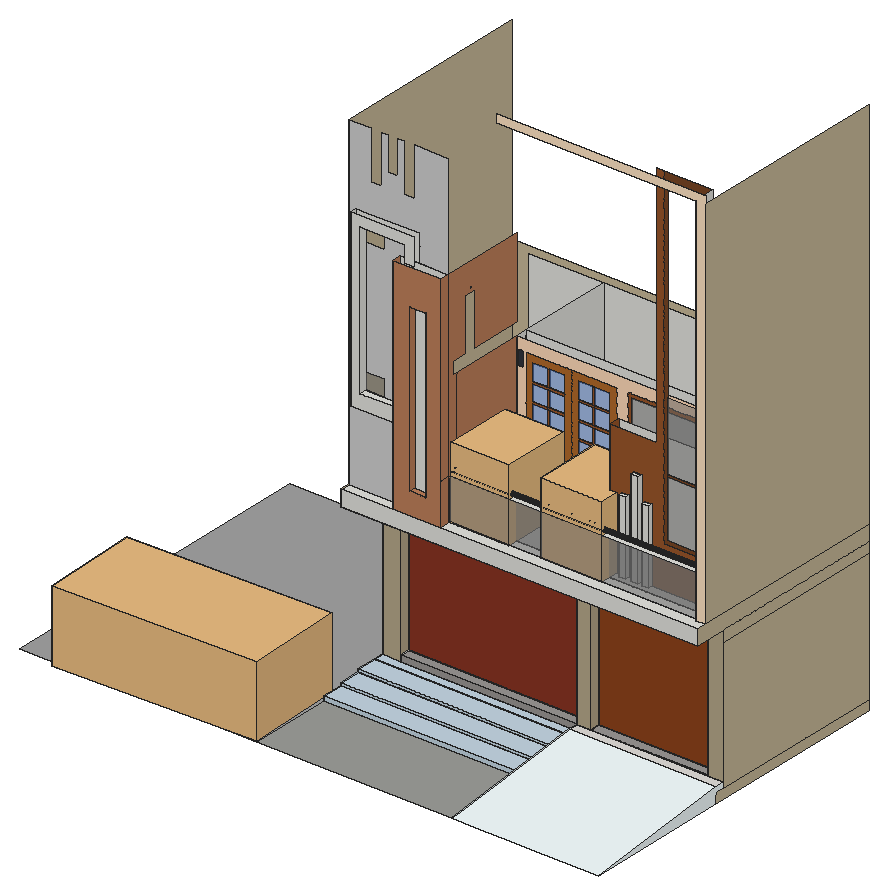
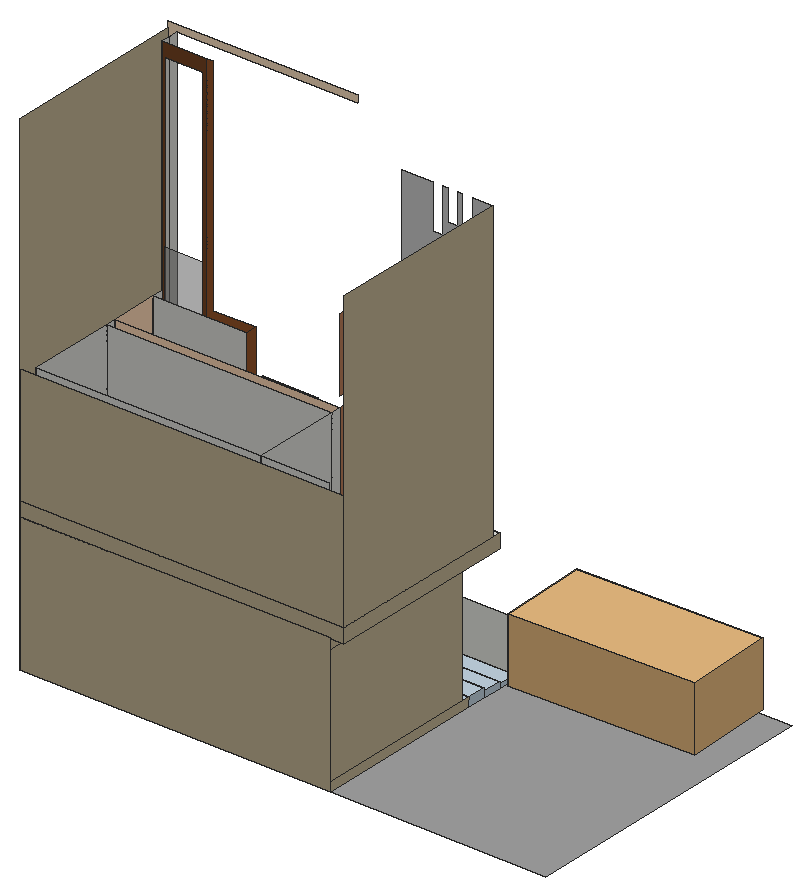
# SketchUp Ruby script. Lengths in inches.
U = 1.inch
M = Sketchup.active_model
def pt(a) = Geom::Point3d.new(a.map { |v| v * U })
def face(e, loops, mat)
  f = e.add_face(loops[0].map { |a| pt(a) })
  loops[1..].each { |l| e.add_face(l.map { |a| pt(a) }).erase! }
  f.material = f.back_material = mat if mat
  f
end
# faces: each face lists its corners as indices into pts; further lists are holes
def faces(e, pts, list, mat = nil) = list.each { |f| face(e, (f[0].is_a?(Array) ? f : [f]).map { |l| l.map { |i| pts[i] } }, mat) }
# xy, xz, yz: faces in a plane at the given z, y or x. An outline is a flat list of corners, or four numbers for a rectangle; further outlines are holes
def ring(l) = l.size == 4 ? [[l[0], l[1]], [l[2], l[1]], [l[2], l[3]], [l[0], l[3]]] : l.each_slice(2).to_a
def flat(e, list, mat, &to3) = list.each { |f| face(e, (f[0].is_a?(Array) ? f : [f]).map { |l| ring(l).map { |u, v| to3.(u, v) } }, mat) }
def xy(e, z, list, mat = nil) = flat(e, list, mat) { |x, y| [x, y, z] }
def xz(e, y, list, mat = nil) = flat(e, list, mat) { |x, z| [x, y, z] }
def yz(e, x, list, mat = nil) = flat(e, list, mat) { |y, z| [x, y, z] }
def lines(e, pts, list) = list.each { |a, b| e.add_line(pt(pts[a]), pt(pts[b])) }
# prism: a flat outline (further loops are holes) pulled along v
def prism(e, loops, v, mat = nil)
  f = face(e, loops, mat); d = Geom::Vector3d.new(v.map { |x| x * U })
  f.pushpull(f.normal.samedirection?(d) ? d.length : -d.length)
end
def box(e, o, s, mat = nil) = prism(e, [[o, [o[0] + s[0], o[1], o[2]], [o[0] + s[0], o[1] + s[1], o[2]], [o[0], o[1] + s[1], o[2]]]], [0, 0, s[2]], mat)
def at(x, y, z, deg = 0) = Geom::Transformation.translation(pt([x, y, z])) * Geom::Transformation.rotation(ORIGIN, Z_AXIS, deg.degrees)
def axes(o, x, y, z) = Geom::Transformation.new([*x, 0, *y, 0, *z, 0, *pt(o).to_a, 1])
def part(name) = M.definitions.add(name)
# library, detail: a bought-in or finely detailed component or shape, given as its bounding box
def library(name, o, s) = part(name).tap { |d| box(d.entities, o, s) }
def detail(e, o, s) = box(e.add_group.entities, o, s)
def put(e, d, t, mat = nil) = e.add_instance(d, t).tap { |i| i.material = mat if mat }
def group(e, t, mat = nil) = e.add_group.tap { |g| g.transformation = t; g.material = mat if mat }.entities
root = M.entities
M.materials.add("[0012_Bisque]").color = [255, 228, 196]
M.materials.add("[0027_PeachPuff]").color = [255, 218, 185]
M.materials.add("[Blinds Weave]1").color = [141, 67, 28]
M.materials.add("[Blinds Wood Light]").color = [137, 52, 35]
M.materials.add("[Cladding Siding White]").color = [207, 207, 207]
M.materials.add("[Concrete Aggregate Smoke]").color = [154, 150, 148]
M.materials.add("[Concrete Block 8x8 Gray]").color = [157, 158, 154]
M.materials.add("[Formica Laminate Dark]").color = [50, 53, 60]
M.materials.add("[Formica Speckled Grey]").color = [94, 105, 111]
M.materials.add("[Pavers Flagstone Gray]").color = [162, 162, 162]
M.materials.add("[Quartz Light Brown]").color = [181, 167, 138]
M.materials.add("[Quartz Light Brown]1").color = [199, 184, 152]
M.materials.add("[Terrazzo Light Blue]").color = [196, 214, 227]
M.materials.add("[Terrazzo Tile Accent]").color = [224, 221, 217]
M.materials.add("[Translucent Glass Blue]").color = [100, 149, 237]
M.materials["[Translucent Glass Blue]"].alpha = 0.5
M.materials.add("[Translucent Glass Gray]").color = [128, 128, 128]
M.materials["[Translucent Glass Gray]"].alpha = 0.5
M.materials.add("[White Subway Tile]").color = [243, 252, 253]
M.materials.add("[Wood Bamboo]").color = [177, 105, 43]
M.materials.add("[Wood Cherry Original]").color = [152, 86, 42]
M.materials.add("[Wood Veneer 01]").color = [120, 70, 37]
M.materials.add("[Wood Veneer 02]").color = [190, 128, 91]
c1 = library("2015 Porsche Macan",[0.14,0.6,0.32],[90.05,184.43,65.58])
c2 = library("chau cay",[-24.34,-109.24,0],[56.46,62.58,79.69])
xy(root,0,[[397.11,0,532.42,22.25],[397.11,22.25,397.41,77.14],[397.41,22.25,532.42,135.01],[218.05,77.14,397.11,96.75],[397.11,77.14,397.41,96.75],
  [218.05,96.75,397.11,116.37],[397.11,96.75,397.41,116.37],[218.05,116.37,397.11,135.01],[397.11,116.37,397.41,135.01],[218.05,135.01,532.42,310.21]])
xy(root,0,[[218.05,0,397.11,77.14]],"[Concrete Block 8x8 Gray]")
xy(root,0,[[0,0,218.05,310.21]],"[Pavers Flagstone Gray]")
xy(root,4.0625,[[218.05,77.14,397.41,96.75]],"[Terrazzo Light Blue]")
xy(root,6.25,[[218.05,96.75,397.41,116.37]],"[Terrazzo Light Blue]")
xy(root,9,[[397.11,135.01,397.41,144.01],[397.41,135.01,532.42,144.01],[235.49,144.01,397.36,152.71],[397.36,144.01,410.16,258.46],[410.16,144.01,517.11,152.71],
  [235.49,152.71,397.36,258.46],[410.16,152.71,517.11,258.46]])
xy(root,9,[[218.05,116.37,397.41,135.01],[218.05,135.01,397.11,144.01]],"[Terrazzo Light Blue]")
xy(root,13.98,[[397.11,135.01,532.42,144.01]],"[Terrazzo Tile Accent]")
xy(root,14.5625,[[235.49,144.01,397.36,152.71],[410.16,144.01,517.11,152.71]],"[Concrete Aggregate Smoke]")
xy(root,129,[[397.36,144.01,410.16,258.46],[235.49,152.71,397.36,258.46],[410.16,152.71,517.11,258.46],[517.11,152.71,532.42,258.46]])
xy(root,129,[[235.49,144.01,397.36,152.71],[410.16,144.01,517.11,152.71]],"[Quartz Light Brown]")
xy(root,139.1875,[[248.73,122.41,246.65,122.68,244.7,123.49,243.03,124.77,241.75,126.4375,240.95,128.38,240.67,130.47,240.95,132.56,241.75,134.5,243.03,136.17,244.7,137.45,246.65,138.26,248.73,138.53,250.82,138.26,252.76,137.45,254.43,136.17,255.72,134.5,256.52,132.56,256.8,130.47,256.52,128.38,255.72,126.4375,254.43,124.77,252.76,123.49,250.82,122.68],[300.55,122.41,298.46,122.68,296.51,123.49,294.84,124.77,293.5625,126.4375,292.76,128.38,292.48,130.47,292.76,132.56,293.5625,134.5,294.84,136.17,296.51,137.45,298.46,138.26,300.55,138.53,302.63,138.26,304.58,137.45,306.25,136.17,307.53,134.5,308.33,132.56,308.61,130.47,308.33,128.38,307.53,126.4375,306.25,124.77,304.58,123.49,302.63,122.68],[364.42,122.41,362.33,122.68,360.39,123.49,358.72,124.77,357.4375,126.4375,356.63,128.38,356.36,130.47,356.63,132.56,357.4375,134.5,358.72,136.17,360.39,137.45,362.33,138.26,364.42,138.53,366.51,138.26,368.45,137.45,370.12,136.17,371.4,134.5,372.21,132.56,372.48,130.47,372.21,128.38,371.4,126.4375,370.12,124.77,368.45,123.49,366.51,122.68],[424.73,122.41,422.65,122.68,420.7,123.49,419.03,124.77,417.75,126.4375,416.95,128.38,416.67,130.47,416.95,132.56,417.75,134.5,419.03,136.17,420.7,137.45,422.65,138.26,424.73,138.53,426.82,138.26,428.76,137.45,430.43,136.17,431.72,134.5,432.52,132.56,432.8,130.47,432.52,128.38,431.72,126.4375,430.43,124.77,428.76,123.49,426.82,122.68],[490.73,122.41,488.65,122.68,486.7,123.49,485.03,124.77,483.75,126.4375,482.95,128.38,482.67,130.47,482.95,132.56,483.75,134.5,485.03,136.17,486.7,137.45,488.65,138.26,490.73,138.53,492.82,138.26,494.76,137.45,496.43,136.17,497.72,134.5,498.52,132.56,498.8,130.47,498.52,128.38,497.72,126.4375,496.43,124.77,494.76,123.49,492.82,122.68],
  [218.05,144.01,532.42,310.21]])
xy(root,139.1875,[[[204.37,113.95,204.37,310.21,218.05,310.21,218.05,144.01,532.42,144.01,532.42,113.95],[248.73,122.41,250.82,122.68,252.76,123.49,254.43,124.77,255.72,126.4375,256.52,128.38,256.8,130.47,256.52,132.56,255.72,134.5,254.43,136.17,252.76,137.45,250.82,138.26,248.73,138.53,246.65,138.26,244.7,137.45,243.03,136.17,241.75,134.5,240.95,132.56,240.67,130.47,240.95,128.38,241.75,126.4375,243.03,124.77,244.7,123.49,246.65,122.68],[490.73,122.41,492.82,122.68,494.76,123.49,496.43,124.77,497.72,126.4375,498.52,128.38,498.8,130.47,498.52,132.56,497.72,134.5,496.43,136.17,494.76,137.45,492.82,138.26,490.73,138.53,488.65,138.26,486.7,137.45,485.03,136.17,483.75,134.5,482.95,132.56,482.67,130.47,482.95,128.38,483.75,126.4375,485.03,124.77,486.7,123.49,488.65,122.68],[300.55,122.41,302.63,122.68,304.58,123.49,306.25,124.77,307.53,126.4375,308.33,128.38,308.61,130.47,308.33,132.56,307.53,134.5,306.25,136.17,304.58,137.45,302.63,138.26,300.55,138.53,298.46,138.26,296.51,137.45,294.84,136.17,293.5625,134.5,292.76,132.56,292.48,130.47,292.76,128.38,293.5625,126.4375,294.84,124.77,296.51,123.49,298.46,122.68],[424.73,122.41,426.82,122.68,428.76,123.49,430.43,124.77,431.72,126.4375,432.52,128.38,432.8,130.47,432.52,132.56,431.72,134.5,430.43,136.17,428.76,137.45,426.82,138.26,424.73,138.53,422.65,138.26,420.7,137.45,419.03,136.17,417.75,134.5,416.95,132.56,416.67,130.47,416.95,128.38,417.75,126.4375,419.03,124.77,420.7,123.49,422.65,122.68],[364.42,122.41,366.51,122.68,368.45,123.49,370.12,124.77,371.4,126.4375,372.21,128.38,372.48,130.47,372.21,132.56,371.4,134.5,370.12,136.17,368.45,137.45,366.51,138.26,364.42,138.53,362.33,138.26,360.39,137.45,358.72,136.17,357.4375,134.5,356.63,132.56,356.36,130.47,356.63,128.38,357.4375,126.4375,358.72,124.77,360.39,123.49,362.33,122.68]]],"[Formica Speckled Grey]")
xy(root,153.375,[[204.37,113.95,251.36,122.95],[251.36,113.95,295.61,122.95],[295.61,113.95,532.42,113.95,532.42,122.95,523.42,122.95,523.42,124.95,295.61,124.95],[204.37,122.95,204.37,310.21,532.42,310.21,532.42,122.95,523.42,122.95,523.42,301.21,227.05,301.21,227.05,122.95],[227.05,122.95,295.61,301.21],
  [295.61,124.95,523.42,132.61],[295.61,132.61,523.42,132.61,523.42,142.27,467.62,142.27,467.62,138.52,460.87,138.52,460.87,142.27,457.85,142.27,457.85,138.52,450.6,138.52,450.6,142.27,446.37,142.27,446.37,138.52,439.62,138.52,439.62,142.27,428.67,142.27,428.67,152.96,523.42,152.96,523.42,201.9,295.61,201.9],[439.62,138.52,446.37,142.27],[450.6,138.52,457.85,142.27],[460.87,138.52,467.62,142.27],
  [428.67,142.27,523.42,152.96],[295.61,201.9,523.42,212.08],[295.61,212.08,523.42,301.21]])
xy(root,173.95,[[267.29,113.95,282.48,119.57]],"[Wood Veneer 02]")
xy(root,191.8125,[[295.61,124.95,523.42,132.61]])
xy(root,221,[[439.62,138.52,446.37,142.27],[460.87,138.52,467.62,142.27]])
xy(root,223.4,[[210.89,116.39,251.36,122.95]])
xy(root,241.625,[[450.6,138.52,457.85,142.27]])
xz(root,77.14,[[218.05,0,397.41,4.0625]],"[Terrazzo Light Blue]")
xz(root,96.75,[[218.05,0,397.41,4.0625]])
xz(root,96.75,[[218.05,4.0625,397.41,6.25]],"[Terrazzo Light Blue]")
xz(root,113.95,[[204.37,139.1875,532.42,153.375]])
xz(root,113.95,[[[251.36,153.375,295.61,358.46],[267.29,173.95,282.48,325.82]]],"[Wood Veneer 02]")
xz(root,116.37,[[218.05,0,397.41,6.25]])
xz(root,116.37,[[218.05,6.25,397.41,9]],"[Terrazzo Light Blue]")
xz(root,116.39,[[210.89,223.4,251.36,223.4,251.36,236.57,219.83,236.51,219.57,373.65,260.41,373.65,260.41,358.46,269.14,358.46,269.14,383.14,210.89,383.14]])
xz(root,119.57,[[267.29,173.95,282.48,325.82]])
xz(root,122.95,[[251.36,153.375,295.61,358.46],[210.89,223.4,210.89,383.14,269.14,383.14,269.14,358.46,260.41,358.46,260.41,373.65,219.57,373.65,219.6,358.46,219.8,251.74,219.57,251.74,219.6,236.55,219.83,236.55,219.83,236.51,237.54,236.55,251.36,236.57,251.36,223.4],[219.83,236.51,237.54,236.55,219.83,236.55],[219.6,236.55,219.83,236.55,219.8,251.74,219.57,251.74]])
xz(root,122.95,[[523.42,153.375,532.42,153.375,532.42,506.6875,340.2,506.6875,340.2,499.5,523.42,499.5]],"[0012_Bisque]")
xz(root,122.95,[[204.37,153.375,251.36,153.375,251.36,223.4,210.89,223.4,210.89,383.14,269.14,383.14,269.14,358.46,295.61,358.46,295.61,454.0625,264.53,454.0625,264.53,410.0625,254.28,410.0625,254.28,454.0625,249.35,454.0625,249.35,423.25,239.66,423.25,239.66,454.0625,234.84,454.0625,234.84,410.0625,224.59,410.0625,224.59,454.0625,204.37,454.0625],[237.54,236.55,251.36,236.57,251.36,358.46,260.41,358.46,260.41,373.65,237.54,373.65,237.54,358.46,219.6,358.46,219.8,251.74,237.54,251.74]],"[Cladding Siding White]")
xz(root,122.95,[[219.83,236.55,237.54,236.55,237.54,251.74,219.8,251.74]],"[Translucent Glass Gray]")
xz(root,124.95,[[295.61,153.375,523.42,191.8125]],"[Translucent Glass Gray]")
xz(root,132.61,[[295.61,153.375,523.42,191.8125]],"[Translucent Glass Gray]")
xz(root,135.01,[[218.05,0,397.11,9],[397.11,0,397.41,9],[397.41,0,532.42,9]])
xz(root,138.52,[[439.62,153.375,446.37,221],[450.6,153.375,457.85,241.625],[460.87,153.375,467.62,221]])
xz(root,142.27,[[439.62,153.375,446.37,221],[450.6,153.375,457.85,241.625],[460.87,153.375,467.62,221]])
xz(root,142.27,[[481.64,195.54,520.01,248.25],[481.64,250.12,520.01,313.87]],"[Translucent Glass Gray]")
xz(root,142.27,[[428.67,153.375,439.62,153.375,439.62,221,446.37,221,446.37,153.375,450.6,153.375,450.6,241.625,457.85,241.625,457.85,153.375,460.87,153.375,460.87,221,467.62,221,467.62,153.375,523.42,153.375,523.42,192.13,478.23,192.13,478.23,499.5,471.875,499.5,471.875,273.375,428.67,273.375]],"[Wood Cherry Original]")
xz(root,142.27,[[[478.23,192.13,523.42,499.5],[481.64,195.54,520.01,486.71]],[481.64,248.25,520.01,250.12]],"[Wood Veneer 01]")
xz(root,144.01,[[397.11,9,397.36,13.98],[397.36,9,410.16,13.98],[410.16,9,517.11,13.98],[517.11,9,532.42,13.98]])
xz(root,144.01,[[235.49,9,397.11,9,397.11,13.98,397.36,13.98,397.36,14.5625,235.49,14.5625],[410.16,13.98,517.11,14.5625]],"[Concrete Aggregate Smoke]")
xz(root,144.01,[[218.05,9,235.49,9,235.49,129,517.11,129,517.11,13.98,532.42,13.98,532.42,139.1875,218.05,139.1875],[397.36,13.98,410.16,129]],"[Quartz Light Brown]")
xz(root,152.71,[[235.49,9,397.36,14.5625],[410.16,9,517.11,14.5625]])
xz(root,152.71,[[410.16,14.5625,517.11,129]],"[Blinds Weave]1")
xz(root,152.71,[[235.49,14.5625,397.36,129]],"[Blinds Wood Light]")
xz(root,152.96,[[428.67,153.375,523.42,273.375]])
xz(root,201.9,[[[295.61,153.375,304.1,153.375,304.1,262.625,387.66,262.625,387.66,153.375,523.42,153.375,523.42,273.375,295.61,273.375],[397.82,197.22,463.76,263.15],[296.63,248.62,301.63,263.18]]],"[0027_PeachPuff]")
xz(root,201.9,[[296.63,248.62,301.63,263.18]],"[Formica Laminate Dark]")
xz(root,201.9,[[310.36,159.64,323.78,175.16],[325.64,159.64,339.62,175.16],[352.14,159.64,365.34,175.16],[367.21,159.64,381.4,175.16],[310.36,177.15,323.78,190.6875],
  [325.64,177.15,339.62,190.6875],[352.14,177.15,365.34,190.6875],[367.21,177.15,381.4,190.6875],[310.36,192.67,323.78,206.5],[325.64,192.67,339.62,206.5],
  [352.14,192.67,365.34,206.5],[367.21,192.67,381.4,206.5],[310.36,208.49,323.78,222.125],[325.64,208.49,339.62,222.125],[352.14,208.49,365.34,222.125],
  [367.21,208.49,381.4,222.125],[310.36,224.11,323.78,238.75],[325.64,224.11,339.62,238.75],[352.14,224.11,365.34,238.75],[367.21,224.11,381.4,238.75],
  [310.36,240.74,323.78,256.36],[325.64,240.74,339.62,256.36],[352.14,240.74,365.34,256.36],[367.21,240.74,381.4,256.36]],"[Translucent Glass Blue]")
xz(root,201.9,[[401.68,201.08,428.25,259.29],[431.53,201.08,459.9,259.29]],"[Translucent Glass Gray]")
xz(root,201.9,[[[304.1,153.375,345.88,262.625],[310.36,159.64,339.62,256.36]],[[345.88,153.375,387.66,262.625],[352.14,159.64,381.4,256.36]]],"[Wood Bamboo]")
xz(root,201.9,[[323.78,159.64,325.64,175.16],[365.34,159.64,367.21,175.16],[310.36,175.16,339.62,177.15],[352.14,175.16,381.4,177.15],[323.78,177.15,325.64,190.6875],
  [365.34,177.15,367.21,190.6875],[310.36,190.6875,339.62,192.67],[352.14,190.6875,381.4,192.67],[323.78,192.67,325.64,206.5],[365.34,192.67,367.21,206.5],
  [[397.82,197.22,463.76,263.15],[401.68,201.08,459.9,259.29]],[428.25,201.08,431.53,259.29],[310.36,206.5,339.62,208.49],[352.14,206.5,381.4,208.49],[323.78,208.49,325.64,222.125],
  [365.34,208.49,367.21,222.125],[310.36,222.125,339.62,224.11],[352.14,222.125,381.4,224.11],[323.78,224.11,325.64,238.75],[365.34,224.11,367.21,238.75],
  [310.36,238.75,339.62,240.74],[352.14,238.75,381.4,240.74],[323.78,240.74,325.64,256.36],[365.34,240.74,367.21,256.36]],"[Wood Cherry Original]")
xz(root,212.08,[[295.61,153.375,523.42,273.375]])
xz(root,258.46,[[235.49,9,397.36,129],[397.36,9,410.16,129],[410.16,9,517.11,129]])
xz(root,301.21,[[227.05,153.375,295.61,273.375],[295.61,153.375,523.42,273.375]])
xz(root,310.21,[[218.05,0,532.42,139.1875],[204.37,139.1875,532.42,153.375],[204.37,153.375,532.42,273.375]],"[Quartz Light Brown]1")
yz(root,204.37,[[113.95,139.1875,310.21,153.375],[122.95,153.375,310.21,454.0625]],"[Quartz Light Brown]1")
yz(root,210.89,[[116.39,223.4,122.95,383.14]])
yz(root,218.05,[[135.01,0,310.21,9],[144.01,9,310.21,129],[144.01,129,310.21,139.1875]],"[Quartz Light Brown]1")
yz(root,218.05,[[77.14,0,96.75,4.0625],[96.75,0,116.37,6.25],[116.37,0,135.01,9]],"[Terrazzo Light Blue]")
yz(root,235.49,[[144.01,9,152.71,14.5625],[152.71,9,258.46,129]])
yz(root,235.49,[[144.01,14.5625,152.71,129]],"[Quartz Light Brown]")
yz(root,251.36,[[116.39,223.4,122.95,236.57]])
yz(root,251.36,[[113.95,153.375,122.95,223.4],[113.95,223.4,116.39,236.57],[113.95,236.57,122.95,358.46]],"[Wood Veneer 02]")
yz(root,267.29,[[113.95,173.95,119.57,325.82]],"[Wood Veneer 02]")
yz(root,282.48,[[113.95,173.95,119.57,325.82]],"[Wood Veneer 02]")
yz(root,295.61,[[124.95,153.375,132.61,191.8125],[201.9,153.375,212.08,273.375],[212.08,153.375,301.21,273.375]])
yz(root,295.61,[[113.95,153.375,122.95,191.8125],[122.95,153.375,124.95,191.8125],[132.61,153.375,201.9,273.375],[113.95,191.8125,122.95,358.46],[[122.95,191.8125,132.61,191.8125,132.61,273.375,128.11,273.375,128.11,284.5625,142.27,284.5625,142.27,332.6875,152.96,332.6875,152.96,284.5625,201.9,284.5625,201.9,358.46,122.95,358.46],[127.92,193.47,127.45,193.53,127.02,193.71,126.64,194,126.35,194.37,126.17,194.81,126.11,195.28,126.17,195.75,126.35,196.18,126.64,196.56,127.02,196.85,127.45,197.03,127.92,197.09,128.39,197.03,128.83,196.85,129.2,196.56,129.49,196.18,129.67,195.75,129.73,195.28,129.67,194.81,129.49,194.37,129.2,194,128.83,193.71,128.39,193.53],[148.83,334.82,148.44,334.87,148.08,335.02,147.77,335.26,147.53,335.57,147.38,335.93,147.33,336.32,147.38,336.7,147.53,337.07,147.77,337.38,148.08,337.62,148.44,337.77,148.83,337.82,149.22,337.77,149.58,337.62,149.89,337.38,150.13,337.07,150.28,336.7,150.33,336.32,150.28,335.93,150.13,335.57,149.89,335.26,149.58,335.02,149.22,334.87]]],"[Wood Veneer 02]")
yz(root,397.11,[[0,0,135.01,13.98,144.01,13.98,144.01,9,135.01,9,135.01,0]],"[White Subway Tile]")
yz(root,397.36,[[144.01,9,152.71,14.5625],[152.71,9,258.46,129]])
yz(root,397.36,[[144.01,14.5625,152.71,129]],"[Quartz Light Brown]")
yz(root,397.41,[[77.14,0,96.75,4.0625],[96.75,0,116.37,6.25],[116.37,0,135.01,9]])
yz(root,410.16,[[144.01,9,152.71,14.5625],[152.71,9,258.46,129]])
yz(root,410.16,[[144.01,14.5625,152.71,129]],"[Quartz Light Brown]")
yz(root,428.67,[[142.27,153.375,152.96,273.375]],"[Wood Cherry Original]")
yz(root,439.62,[[138.52,153.375,142.27,221]])
yz(root,446.37,[[138.52,153.375,142.27,221]])
yz(root,450.6,[[138.52,153.375,142.27,241.625]])
yz(root,457.85,[[138.52,153.375,142.27,241.625]])
yz(root,460.87,[[138.52,153.375,142.27,221]])
yz(root,467.62,[[138.52,153.375,142.27,221]])
yz(root,517.11,[[144.01,9,152.71,14.5625],[152.71,9,258.46,129]])
yz(root,517.11,[[144.01,14.5625,152.71,129]],"[Quartz Light Brown]")
yz(root,523.42,[[122.95,153.375,124.95,191.8125],[124.95,153.375,132.61,191.8125],[132.61,153.375,142.27,499.5],[142.27,153.375,152.96,273.375],[201.9,153.375,212.08,273.375],
  [212.08,153.375,301.21,273.375],[[122.95,191.8125,132.61,499.5],[127.92,193.47,128.39,193.53,128.83,193.71,129.2,194,129.49,194.37,129.67,194.81,129.73,195.28,129.67,195.75,129.49,196.18,129.2,196.56,128.83,196.85,128.39,197.03,127.92,197.09,127.45,197.03,127.02,196.85,126.64,196.56,126.35,196.18,126.17,195.75,126.11,195.28,126.17,194.81,126.35,194.37,126.64,194,127.02,193.71,127.45,193.53]],[127.92,193.47,128.39,193.53,128.83,193.71,129.2,194,129.49,194.37,129.67,194.81,129.73,195.28,129.67,195.75,129.49,196.18,129.2,196.56,128.83,196.85,128.39,197.03,127.92,197.09,127.45,197.03,127.02,196.85,126.64,196.56,126.35,196.18,126.17,195.75,126.11,195.28,126.17,194.81,126.35,194.37,126.64,194,127.02,193.71,127.45,193.53]])
yz(root,523.42,[[152.96,153.375,201.9,273.375]],"[0027_PeachPuff]")
yz(root,532.42,[[135.01,0,310.21,9],[144.01,9,310.21,129],[144.01,129,310.21,139.1875],[113.95,139.1875,310.21,153.375],[122.95,153.375,310.21,499.5]],"[Quartz Light Brown]1")
yz(root,532.42,[[0,0,135.01,0,135.01,9,144.01,9,144.01,13.98,135.01,13.98]],"[White Subway Tile]")
p = [[397.11,135.01,13.98],[397.11,0,0],[419.47,0,0],[443.01,0,0],[466.56,0,0],[532.42,0,0],
  [532.42,135.01,13.98],[523.42,127.45,193.53],[523.42,127.02,193.71],[295.61,127.02,193.71],[295.61,127.45,193.53],[523.42,127.92,193.47],
  [295.61,127.92,193.47],[523.42,128.39,193.53],[295.61,128.39,193.53],[523.42,128.83,193.71],[295.61,128.83,193.71],[523.42,126.64,194],
  [295.61,126.64,194],[523.42,129.2,194],[295.61,129.2,194],[523.42,126.35,194.37],[295.61,126.35,194.37],[523.42,129.49,194.37],
  [295.61,129.49,194.37],[523.42,126.17,194.81],[295.61,126.17,194.81],[523.42,129.67,194.81],[295.61,129.67,194.81],[523.42,126.11,195.28],
  [295.61,126.11,195.28],[523.42,129.73,195.28],[295.61,129.73,195.28],[523.42,126.17,195.75],[295.61,126.17,195.75],[523.42,129.67,195.75],
  [295.61,129.67,195.75],[523.42,126.35,196.18],[295.61,126.35,196.18],[523.42,129.49,196.18],[295.61,129.49,196.18],[523.42,126.64,196.56],
  [295.61,126.64,196.56],[523.42,129.2,196.56],[295.61,129.2,196.56],[523.42,127.02,196.85],[295.61,127.02,196.85],[523.42,128.83,196.85],
  [295.61,128.83,196.85],[523.42,127.45,197.03],[295.61,127.45,197.03],[523.42,128.39,197.03],[295.61,128.39,197.03],[523.42,127.92,197.09],
  [295.61,127.92,197.09],[219.6,122.95,358.46],[219.57,122.95,373.65],[219.57,116.39,373.65],[219.83,116.39,236.51],[219.83,122.95,236.51],
  [219.83,122.95,236.55],[219.8,122.95,251.74],[237.54,122.95,236.55],[251.36,116.39,236.57],[251.36,122.95,236.57],[235.49,152.71,129],
  [218.05,152.71,129],[235.49,258.46,129],[235.49,267.46,129],[397.36,258.46,129],[397.36,267.46,129],[410.16,258.46,129],
  [410.16,267.46,129]]
faces(root,p,[[0,1,2,3,4,5,6]],"[White Subway Tile]")
faces(root,p,[[7,8,9,10],[11,7,10,12],[13,11,12,14],[15,13,14,16],[8,17,18,9],[19,15,16,20],[17,21,22,18],[23,19,20,24],
  [21,25,26,22],[27,23,24,28],[25,29,30,26],[31,27,28,32],[29,33,34,30],[35,31,32,36],[33,37,38,34],[39,35,36,40],
  [37,41,42,38],[43,39,40,44],[41,45,46,42],[47,43,44,48],[45,49,50,46],[51,47,48,52],[49,53,54,50],[53,51,52,54]],"[Terrazzo Light Blue]")
faces(root,p,[[55,56,57,58,59,60,61],[62,59,58,63,64]])
lines(root,p,[[65,66],[67,68],[69,70],[71,72]])
put(root,c1,at(218.05,0,0,91.7))
put(root,c2,axes([317.83,234.1875,153.375],[1,0,0],[0,1,0],[0,0,0.83]))
put(root,c2,axes([403.34,234.1875,153.375],[1,0,0],[0,1,0],[0,0,0.83]))
